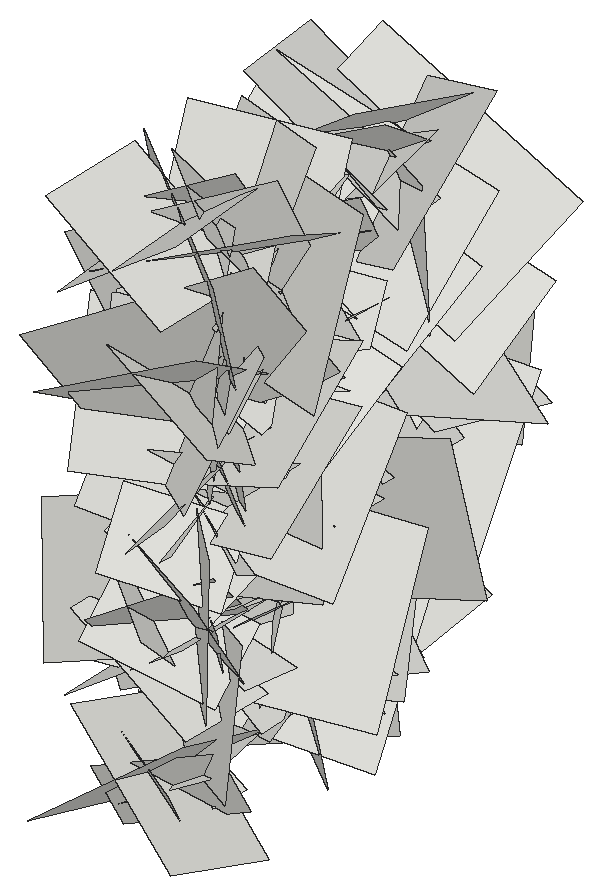
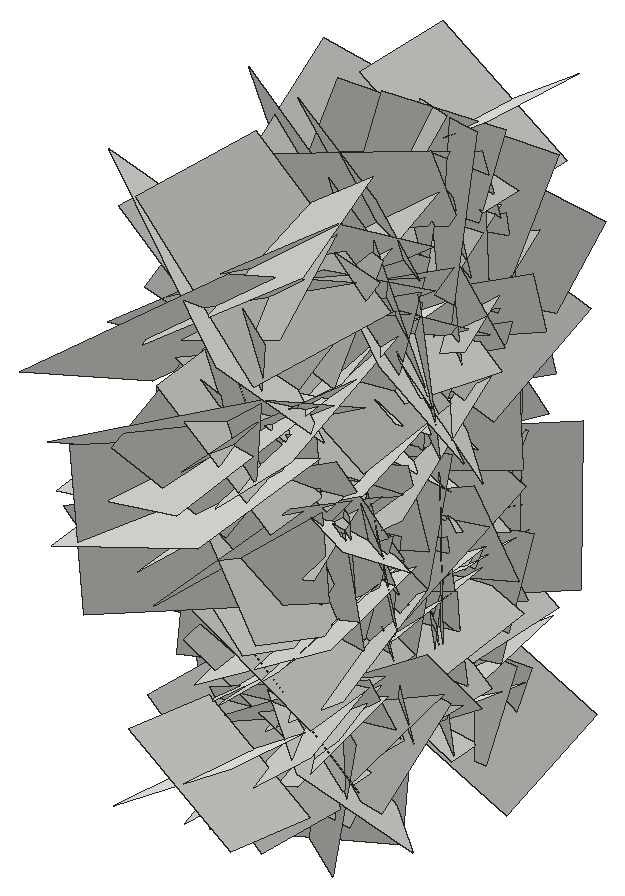
# SketchUp Ruby script. Lengths in inches.
U = 1.inch
M = Sketchup.active_model
def pt(a) = Geom::Point3d.new(a.map { |v| v * U })
def face(e, loops, mat)
  f = e.add_face(loops[0].map { |a| pt(a) })
  loops[1..].each { |l| e.add_face(l.map { |a| pt(a) }).erase! }
  f.material = f.back_material = mat if mat
  f
end
# faces: each face lists its corners as indices into pts; further lists are holes
def faces(e, pts, list, mat = nil) = list.each { |f| face(e, (f[0].is_a?(Array) ? f : [f]).map { |l| l.map { |i| pts[i] } }, mat) }
# xy, xz, yz: faces in a plane at the given z, y or x. An outline is a flat list of corners, or four numbers for a rectangle; further outlines are holes
def ring(l) = l.size == 4 ? [[l[0], l[1]], [l[2], l[1]], [l[2], l[3]], [l[0], l[3]]] : l.each_slice(2).to_a
def flat(e, list, mat, &to3) = list.each { |f| face(e, (f[0].is_a?(Array) ? f : [f]).map { |l| ring(l).map { |u, v| to3.(u, v) } }, mat) }
def xy(e, z, list, mat = nil) = flat(e, list, mat) { |x, y| [x, y, z] }
def xz(e, y, list, mat = nil) = flat(e, list, mat) { |x, z| [x, y, z] }
def yz(e, x, list, mat = nil) = flat(e, list, mat) { |y, z| [x, y, z] }
def lines(e, pts, list) = list.each { |a, b| e.add_line(pt(pts[a]), pt(pts[b])) }
# prism: a flat outline (further loops are holes) pulled along v
def prism(e, loops, v, mat = nil)
  f = face(e, loops, mat); d = Geom::Vector3d.new(v.map { |x| x * U })
  f.pushpull(f.normal.samedirection?(d) ? d.length : -d.length)
end
def box(e, o, s, mat = nil) = prism(e, [[o, [o[0] + s[0], o[1], o[2]], [o[0] + s[0], o[1] + s[1], o[2]], [o[0], o[1] + s[1], o[2]]]], [0, 0, s[2]], mat)
def at(x, y, z, deg = 0) = Geom::Transformation.translation(pt([x, y, z])) * Geom::Transformation.rotation(ORIGIN, Z_AXIS, deg.degrees)
def axes(o, x, y, z) = Geom::Transformation.new([*x, 0, *y, 0, *z, 0, *pt(o).to_a, 1])
def part(name) = M.definitions.add(name)
# library, detail: a bought-in or finely detailed component or shape, given as its bounding box
def library(name, o, s) = part(name).tap { |d| box(d.entities, o, s) }
def detail(e, o, s) = box(e.add_group.entities, o, s)
def put(e, d, t, mat = nil) = e.add_instance(d, t).tap { |i| i.material = mat if mat }
def group(e, t, mat = nil) = e.add_group.tap { |g| g.transformation = t; g.material = mat if mat }.entities
root = M.entities
c1 = part("Component\#6")
p = [[0.01,0,0],[0,3.24,4.54],[4.32,3.24,4.54],[4.33,0,0]]
faces(c1.entities,p,[[0,1,2,3]])
put(root,c1,axes([38.11,185.4,30.76],[0.02152,-0.00963,-1.2106],[0.23963,-1.18945,0.01326],[-1.26071,-0.22625,-0.01814]))
put(root,c1,axes([34.14,183.74,37.84],[0.08456,-0.37494,0.46177],[-0.03825,0.46199,0.38136],[0.62935,0.07846,-0.03886]))
put(root,c1,axes([34.14,188.62,32.29],[-0.0866,-0.74743,0.19758],[-0.06186,0.20408,0.74787],[0.81715,-0.06376,0.07755]))
put(root,c1,axes([34.14,184.65,28.76],[0.04824,-0.62434,-0.28052],[-0.09786,-0.28417,0.61748],[0.7189,0.00321,0.10288]))
put(root,c1,axes([38.11,186.48,30.64],[-0.03295,0.70699,0.47041],[-0.18441,0.45544,-0.69599],[-0.88105,-0.12176,0.12808]))
put(root,c1,axes([38.11,180.55,24.45],[-0.04702,0.95483,-0.28451],[0.08229,-0.28062,-0.95386],[-1.05288,-0.06457,-0.06184]))
put(root,c1,axes([38.11,184.8,33.37],[-0.19651,0.19461,-0.78555],[0.01158,-0.80522,-0.20206],[-0.85778,-0.05545,0.17724]))
put(root,c1,axes([38.11,181.12,36.49],[0.0887,0.85058,-0.45713],[-0.14057,-0.44437,-0.85112],[-1.01388,0.13603,0.07801]))
put(root,c1,axes([34.14,182.11,23.57],[-0.01533,0.32032,-0.55846],[0.07998,-0.55391,-0.31966],[0.67773,0.07262,0.02509]))
put(root,c1,axes([34.14,186.27,36.66],[-0.23271,0.08267,-1.0169],[-0.17131,-1.02986,-0.04883],[1.06781,-0.14721,-0.22945]))
put(root,c1,axes([34.14,181.88,29.24],[0.0732,0.47057,-0.46808],[-0.06498,-0.46407,-0.47558],[0.70054,-0.09222,0.00479]))
put(root,c1,axes([34.14,188.01,25.87],[-0.18323,0.88768,-0.1275],[-0.06793,-0.14175,-0.89995],[0.94816,0.16139,-0.08912]))
put(root,c1,axes([38.11,186.85,26],[-0.04759,0.74401,-0.43208],[-0.09551,-0.43435,-0.73856],[-0.90698,0.0067,0.10045]))
put(root,c1,axes([38.11,182.62,33.52],[0.16113,0.63843,0.91206],[0.00988,0.91976,-0.64538],[-1.18006,0.09488,0.11913]))
put(root,c1,axes([34.14,188.3,31.13],[-0.1103,-0.11339,-0.88165],[-0.13763,-0.87621,0.12802],[0.93214,-0.14279,-0.08543]))
put(root,c1,axes([38.11,182.86,27.86],[-0.00866,0.87216,-0.09866],[-0.12421,-0.09886,-0.86427],[-0.92206,0.00513,0.11735]))
put(root,c1,axes([34.14,188.48,31.6],[0.00806,0.51701,-0.38199],[0.06142,-0.38101,-0.51453],[0.67861,0.02834,0.0511]))
put(root,c1,axes([34.14,189.49,31],[-0.19159,0.03614,-0.77666],[0.1449,-0.78347,-0.06827],[0.81131,0.14846,-0.17121]))
put(root,c1,axes([38.11,186.8,27.07],[0.11611,-1.02809,0.5245],[0.14127,0.5346,1.02006],[-1.21522,-0.03608,0.16869]))
put(root,c1,axes([34.14,181.75,22.9],[0.07496,0.59984,0.04506],[0.05269,0.03939,-0.60235],[0.63545,-0.07402,0.04463]))
put(root,c1,axes([38.11,190.89,25.45],[0.07637,-0.93381,0.1535],[-0.06656,0.14888,0.93522],[-1.00091,-0.08115,-0.05048]))
put(root,c1,axes([38.11,189.24,21.76],[-0.15995,-0.688,0.38857],[0.02017,0.39231,0.70202],[-0.83731,0.14088,-0.05731]))
put(root,c1,axes([34.14,186.9,33.68],[-0.12726,-0.80704,-0.07778],[0.05104,-0.08559,0.81372],[0.85791,-0.11462,-0.05995]))
put(root,c1,axes([34.14,183.3,35.54],[0.06853,-0.0517,0.64839],[0.02911,0.65122,0.04919],[0.68886,-0.02238,-0.06659]))
put(root,c1,axes([38.11,182.91,34.72],[0.14912,-0.41506,0.98502],[0.044,0.99488,0.41329],[-1.13217,-0.016,0.1458]))
put(root,c1,axes([38.11,191.48,24.4],[0.24044,-0.84726,-0.84182],[0.11443,-0.83882,0.87332],[-1.26085,-0.2377,-0.08127]))
put(root,c1,axes([34.14,194.3125,23.26],[-0.02367,-0.75059,-0.08188],[0.02978,-0.08269,0.75031],[0.79979,-0.01914,-0.03036]))
put(root,c1,axes([38.11,189.58,22.99],[0.08755,-0.94666,0.34405],[0.04779,0.34833,0.94763],[-1.06661,-0.0621,0.0707]))
put(root,c1,axes([38.11,183.5625,38.07],[-0.03427,-0.86867,-0.02883],[0.01016,-0.0292,0.8692],[-0.92124,0.03199,0.01066]))
put(root,c1,axes([34.14,186.98,23.44],[-0.07046,0.41434,0.63319],[0.10971,0.63463,-0.40442],[0.79457,-0.05088,0.11199]))
put(root,c1,axes([38.11,186.99,20.26],[-0.04681,-0.17583,0.86867],[0.05724,0.86759,0.17835],[-0.93771,0.06173,-0.03248]))
put(root,c1,axes([34.14,182.78,23.92],[-0.06221,-0.24398,0.83625],[-0.07047,0.83695,0.23952],[0.92069,0.04758,0.07484]))
put(root,c1,axes([38.11,187.32,34.27],[-0.05201,-0.4187,0.7383],[0.02779,0.73844,0.42051],[-0.89926,0.04704,-0.0297]))
put(root,c1,axes([34.14,187.84,31.26],[0.01205,0.8882,0.30464],[-0.22592,0.29915,-0.86424],[0.96935,0.05868,-0.20521]))
put(root,c1,axes([34.14,187.61,26.86],[-0.07932,-0.16974,-0.83453],[-0.0041,-0.83766,0.17072],[0.9027,-0.01872,-0.07255]))
put(root,c1,axes([34.14,184.84,39.1],[0.02023,-0.20369,-0.6632],[0.11732,-0.65406,0.20407],[0.72599,0.11137,-0.0145]))
put(root,c1,axes([38.11,180.54,27.52],[-0.00647,0.86334,-0.00303],[0.00368,-0.003,-0.86336],[-0.91514,-0.00612,-0.00345]))
put(root,c1,axes([38.11,189.53,40.3125],[0.07096,0.70634,-0.4758],[-0.12627,-0.46481,-0.70678],[-0.89387,0.12173,0.06207]))
put(root,c1,axes([38.11,192.58,32.17],[-0.11188,-0.86522,-0.03173],[0.14554,-0.04829,0.85998],[-0.90613,0.09907,0.14204]))
put(root,c1,axes([38.11,185.86,28.71],[0.06844,0.29244,0.76285],[-0.17475,0.75415,-0.27515],[-0.84819,-0.13178,0.11824]))
put(root,c1,axes([34.14,188.23,41.22],[-0.26749,1.02168,-0.17372],[0.00845,-0.17688,-1.05183],[1.0985,0.25014,-0.03421]))
put(root,c1,axes([38.11,187.08,35.11],[0.23629,-0.52338,-1.02054],[0.13084,-1.02265,0.55142],[-1.20867,-0.21302,-0.13982]))
put(root,c1,axes([34.14,187.74,23.43],[-0.08523,-0.9506,0.05636],[-0.09187,0.06363,0.94959],[1.00521,-0.07479,0.09156]))
put(root,c1,axes([34.14,184.52,38.07],[-0.06477,0.36641,0.7198],[0.11209,0.71927,-0.35717],[0.84878,-0.06703,0.10209]))
put(root,c1,axes([34.14,184.92,37.05],[0.01613,-0.13323,-0.78421],[0.01491,-0.78419,0.1335],[0.84304,0.01642,0.01265]))
put(root,c1,axes([38.11,184.92,37.05],[-0.01613,-0.13323,-0.78421],[-0.01491,-0.78419,0.1335],[-0.84304,0.01642,0.01265]))
put(root,c1,axes([38.11,184.52,38.07],[0.06477,0.36641,0.7198],[-0.11209,0.71927,-0.35717],[-0.84878,-0.06703,0.10209]))
put(root,c1,axes([38.11,187.74,23.43],[0.08523,-0.9506,0.05636],[0.09187,0.06363,0.94959],[-1.00521,-0.07479,0.09156]))
put(root,c1,axes([34.14,187.08,35.11],[-0.23629,-0.52338,-1.02054],[-0.13084,-1.02265,0.55142],[1.20867,-0.21302,-0.13982]))
put(root,c1,axes([38.11,188.23,41.22],[0.26749,1.02168,-0.17372],[-0.00845,-0.17688,-1.05183],[-1.0985,0.25014,-0.03421]))
put(root,c1,axes([34.14,185.86,28.71],[-0.06844,0.29244,0.76285],[0.17475,0.75415,-0.27515],[0.84819,-0.13178,0.11824]))
put(root,c1,axes([34.14,192.58,32.17],[0.11188,-0.86522,-0.03173],[-0.14554,-0.04829,0.85998],[0.90613,0.09907,0.14204]))
put(root,c1,axes([34.14,189.53,40.3125],[-0.07096,0.70634,-0.4758],[0.12627,-0.46481,-0.70678],[0.89387,0.12173,0.06207]))
put(root,c1,axes([34.14,180.54,27.52],[0.00647,0.86334,-0.00303],[-0.00368,-0.003,-0.86336],[0.91514,-0.00612,-0.00345]))
put(root,c1,axes([38.11,184.84,39.1],[-0.02023,-0.20369,-0.6632],[-0.11732,-0.65406,0.20407],[-0.72599,0.11137,-0.0145]))
put(root,c1,axes([38.11,187.61,26.86],[0.07932,-0.16974,-0.83453],[0.0041,-0.83766,0.17072],[-0.9027,-0.01872,-0.07255]))
put(root,c1,axes([38.11,187.84,31.26],[-0.01205,0.8882,0.30464],[0.22592,0.29915,-0.86424],[-0.96935,0.05868,-0.20521]))
put(root,c1,axes([34.14,187.32,34.27],[0.05201,-0.4187,0.7383],[-0.02779,0.73844,0.42051],[0.89926,0.04704,-0.0297]))
put(root,c1,axes([38.11,182.78,23.92],[0.06221,-0.24398,0.83625],[0.07047,0.83695,0.23952],[-0.92069,0.04758,0.07484]))
put(root,c1,axes([34.14,186.99,20.26],[0.04681,-0.17583,0.86867],[-0.05724,0.86759,0.17835],[0.93771,0.06173,-0.03248]))
put(root,c1,axes([38.11,186.98,23.44],[0.07046,0.41434,0.63319],[-0.10971,0.63463,-0.40442],[-0.79457,-0.05088,0.11199]))
put(root,c1,axes([34.14,183.5625,38.07],[0.03427,-0.86867,-0.02883],[-0.01016,-0.0292,0.8692],[0.92124,0.03199,0.01066]))
put(root,c1,axes([34.14,189.58,22.99],[-0.08755,-0.94666,0.34405],[-0.04779,0.34833,0.94763],[1.06661,-0.0621,0.0707]))
put(root,c1,axes([38.11,194.3125,23.26],[0.02367,-0.75059,-0.08188],[-0.02978,-0.08269,0.75031],[-0.79979,-0.01914,-0.03036]))
put(root,c1,axes([34.14,191.48,24.4],[-0.24044,-0.84726,-0.84182],[-0.11443,-0.83882,0.87332],[1.26085,-0.2377,-0.08127]))
put(root,c1,axes([34.14,182.91,34.72],[-0.14912,-0.41506,0.98502],[-0.044,0.99488,0.41329],[1.13217,-0.016,0.1458]))
put(root,c1,axes([38.11,183.3,35.54],[-0.06853,-0.0517,0.64839],[-0.02911,0.65122,0.04919],[-0.68886,-0.02238,-0.06659]))
put(root,c1,axes([38.11,186.9,33.68],[0.12726,-0.80704,-0.07778],[-0.05104,-0.08559,0.81372],[-0.85791,-0.11462,-0.05995]))
put(root,c1,axes([34.14,189.24,21.76],[0.15995,-0.688,0.38857],[-0.02017,0.39231,0.70202],[0.83731,0.14088,-0.05731]))
put(root,c1,axes([34.14,190.89,25.45],[-0.07637,-0.93381,0.1535],[0.06656,0.14888,0.93522],[1.00091,-0.08115,-0.05048]))
put(root,c1,axes([38.11,181.75,22.9],[-0.07496,0.59984,0.04506],[-0.05269,0.03939,-0.60235],[-0.63545,-0.07402,0.04463]))
put(root,c1,axes([34.14,186.8,27.07],[-0.11611,-1.02809,0.5245],[-0.14127,0.5346,1.02006],[1.21522,-0.03608,0.16869]))
put(root,c1,axes([38.11,189.49,31],[0.19159,0.03614,-0.77666],[-0.1449,-0.78347,-0.06827],[-0.81131,0.14846,-0.17121]))
put(root,c1,axes([38.11,188.48,31.6],[-0.00806,0.51701,-0.38199],[-0.06142,-0.38101,-0.51453],[-0.67861,0.02834,0.0511]))
put(root,c1,axes([34.14,182.86,27.86],[0.00866,0.87216,-0.09866],[0.12421,-0.09886,-0.86427],[0.92206,0.00513,0.11735]))
put(root,c1,axes([38.11,188.3,31.13],[0.1103,-0.11339,-0.88165],[0.13763,-0.87621,0.12802],[-0.93214,-0.14279,-0.08543]))
put(root,c1,axes([34.14,182.62,33.52],[-0.16113,0.63843,0.91206],[-0.00988,0.91976,-0.64538],[1.18006,0.09488,0.11913]))
put(root,c1,axes([34.14,186.85,26],[0.04759,0.74401,-0.43208],[0.09551,-0.43435,-0.73856],[0.90698,0.0067,0.10045]))
put(root,c1,axes([38.11,188.01,25.87],[0.18323,0.88768,-0.1275],[0.06793,-0.14175,-0.89995],[-0.94816,0.16139,-0.08912]))
put(root,c1,axes([38.11,181.88,29.24],[-0.0732,0.47057,-0.46808],[0.06498,-0.46407,-0.47558],[-0.70054,-0.09222,0.00479]))
put(root,c1,axes([38.11,186.27,36.66],[0.23271,0.08267,-1.0169],[0.17131,-1.02986,-0.04883],[-1.06781,-0.14721,-0.22945]))
put(root,c1,axes([38.11,182.11,23.57],[0.01533,0.32032,-0.55846],[-0.07998,-0.55391,-0.31966],[-0.67773,0.07262,0.02509]))
put(root,c1,axes([34.14,181.12,36.49],[-0.0887,0.85058,-0.45713],[0.14057,-0.44437,-0.85112],[1.01388,0.13603,0.07801]))
put(root,c1,axes([34.14,184.8,33.37],[0.19651,0.19461,-0.78555],[-0.01158,-0.80522,-0.20206],[0.85778,-0.05545,0.17724]))
put(root,c1,axes([34.14,180.55,24.45],[0.04702,0.95483,-0.28451],[-0.08229,-0.28062,-0.95386],[1.05288,-0.06457,-0.06184]))
put(root,c1,axes([34.14,186.48,30.64],[0.03295,0.70699,0.47041],[0.18441,0.45544,-0.69599],[0.88105,-0.12176,0.12808]))
put(root,c1,axes([38.11,184.65,28.76],[-0.04824,-0.62434,-0.28052],[0.09786,-0.28417,0.61748],[-0.7189,0.00321,0.10288]))
put(root,c1,axes([38.11,188.62,32.29],[0.0866,-0.74743,0.19758],[0.06186,0.20408,0.74787],[-0.81715,-0.06376,0.07755]))
put(root,c1,axes([38.11,183.74,37.84],[-0.08456,-0.37494,0.46177],[0.03825,0.46199,0.38136],[-0.62935,0.07846,-0.03886]))
put(root,c1,axes([34.14,185.4,30.76],[-0.02152,-0.00963,-1.2106],[-0.23963,-1.18945,0.01326],[1.26071,-0.22625,-0.01814]))
put(root,c1,axes([34.14,187.18,35.87],[-0.21905,1.32848,-0.23139],[-0.18572,-0.25856,-1.32798],[1.41727,0.17144,-0.20979]))
put(root,c1,axes([38.11,188.41,35.3125],[-0.03073,0.48255,0.4704],[0.10717,0.46862,-0.47449],[-0.70624,0.05011,-0.09248]))
put(root,c1,axes([38.11,183.98,26.9],[0.15473,-0.64925,-0.29626],[-0.07231,-0.3137,0.65387],[-0.75301,-0.10329,-0.12366]))
put(root,c1,axes([38.11,183.4375,30.23],[0.10865,-0.24445,0.66529],[-0.00738,0.67183,0.24793],[-0.75127,-0.04195,0.09378]))
put(root,c1,axes([38.11,185.35,37.93],[0.06077,0.5182,0.40006],[-0.00909,0.40215,-0.51968],[-0.69387,0.04012,0.04185]))
put(root,c1,axes([34.14,182.41,31.86],[-0.21699,-0.67676,1.03332],[0.0082,1.04669,0.68705],[1.3093,-0.11872,0.16695]))
put(root,c1,axes([34.14,181.64,30.57],[0.02444,0.48831,-0.77146],[0.19424,-0.75848,-0.47462],[0.9481,0.1428,0.11713]))
put(root,c1,axes([34.14,184.85,32.98],[-0.15473,1.07562,-0.16592],[0.16403,-0.14519,-1.07739],[1.14193,0.1666,0.13228]))
put(root,c1,axes([38.11,179.78,31.84],[0.01485,0.68647,0.23212],[0.1576,0.2245,-0.67291],[-0.75179,0.06062,-0.13648]))
put(root,c1,axes([38.11,188.93,38.32],[0.06934,0.59373,0.25],[-0.00198,0.25145,-0.59671],[-0.68287,0.05956,0.02711]))
put(root,c1,axes([38.11,193.29,29.97],[-0.02765,-0.60791,0.13872],[0.08921,0.13414,0.60366],[-0.6549,0.04394,0.07638]))
put(root,c1,axes([34.14,189.07,22.99],[0.09993,-0.91741,-0.05408],[0.10319,-0.04408,0.91762],[0.96866,0.09934,-0.09218]))
put(root,c1,axes([34.14,185.63,37.94],[-0.10296,1.07287,0.66666],[-0.13207,0.65722,-1.07584],[1.33238,0.14805,-0.05512]))
put(root,c1,axes([34.14,185.55,26.35],[0.05433,-0.24183,-1.04679],[-0.06418,-1.04696,0.23891],[1.13701,-0.04754,0.0635]))
put(root,c1,axes([38.11,186.02,29.02],[0.12909,0.32312,-0.64935],[0.06195,-0.66067,-0.31779],[-0.76632,0.00102,-0.13508]))
put(root,c1,axes([34.14,190.19,31.82],[0.07854,-1.04848,0.11995],[-0.05802,0.11627,1.05008],[1.11713,0.07975,0.0461]))
put(root,c1,axes([38.11,188.83,29.07],[0.04972,0.59189,0.16701],[0.02122,0.16593,-0.59371],[-0.65156,0.05057,-0.00659]))
put(root,c1,axes([34.14,185.29,39.56],[0.11827,0.82487,-0.51088],[0.03346,-0.51706,-0.82795],[1.02793,-0.07808,0.08573]))
put(root,c1,axes([34.14,186.92,28.87],[0.11772,1.08189,-0.3436],[-0.18933,-0.32428,-1.0788],[1.18826,-0.15885,-0.13785]))
put(root,c1,axes([38.11,191.45,35.51],[0.13227,0.51495,-0.41011],[0.00116,-0.41758,-0.52399],[-0.6978,0.09692,-0.07861]))
put(root,c1,axes([38.11,183.51,30.36],[0.10644,-0.42009,-0.4575],[-0.01901,-0.46521,0.42323],[-0.65811,-0.0545,-0.08622]))
put(root,c1,axes([34.14,184.16,23.6],[0.00632,0.19994,1.20323],[-0.15077,1.19515,-0.1979],[1.28409,0.13934,-0.02916]))
put(root,c1,axes([34.14,189.26,31.29],[0.07003,-0.18149,-1.00879],[0.05402,-1.00905,0.18487],[1.08514,0.06195,0.0559]))
put(root,c1,axes([38.11,191.07,24.72],[0.08022,-0.60182,-0.03468],[0.03515,-0.03074,0.60586],[-0.63802,-0.07736,0.02902]))
put(root,c1,axes([34.14,187.65,25.55],[0.14301,-0.32766,0.90945],[0.11586,0.91755,0.31436],[1.01811,-0.05839,-0.16352]))
put(root,c1,axes([34.14,192.86,38.11],[0.10772,-0.0541,-1.0459],[0.04447,-1.04976,0.05837],[1.10925,0.04734,0.09923]))
put(root,c1,axes([38.11,188.74,27.6],[0.13014,-0.45431,-0.37588],[0.00674,-0.3829,0.46487],[-0.62498,-0.09873,-0.07326]))
put(root,c1,axes([34.14,181.98,27.65],[0.03848,-0.07343,1.06513],[0.13392,1.05855,0.06867],[1.12376,-0.12364,-0.04466]))
put(root,c1,axes([34.14,182.88,33.98],[0.05541,0.90127,0.55592],[0.17138,0.54328,-0.89597],[1.1093,-0.12895,0.11065]))
put(root,c1,axes([34.14,190.1,29],[0.15352,-0.05709,1.12322],[-0.06907,1.13017,0.06585],[1.19015,0.07295,-0.14107]))
put(root,c1,axes([34.14,185.59,36.56],[0.07365,1.00309,0.56692],[0.00038,0.56794,-1.00493],[1.22135,-0.06067,-0.03387]))
put(root,c1,axes([34.14,194.96,38.36],[-0.08597,-0.96025,-0.92678],[-0.03419,-0.92681,0.9631],[1.41421,-0.08078,-0.03305]))
put(root,c1,axes([34.14,188.57,34.3],[-0.02784,1.05016,0.5271],[0.1514,0.52617,-1.0412],[1.23628,-0.04079,0.13938]))
put(root,c1,axes([34.14,186.91,28.91],[-0.08475,0.77289,1.06783],[0.0494,1.07079,-0.77154],[1.39641,0.00903,0.0921]))
put(root,c1,axes([34.14,187.29,32.09],[-0.03087,-0.89426,-0.74249],[0.26998,-0.72958,0.86873],[1.20212,0.14089,-0.21417]))
put(root,c1,axes([34.14,190.5,33.59],[0.11278,1.05886,-0.21225],[0.21462,-0.22906,-1.04119],[1.12442,-0.06248,0.22002]))
put(root,c1,axes([34.14,184.99,36.41],[0.13687,-0.99381,0.45239],[0.15227,0.46704,0.985],[1.14738,0.05657,-0.18469]))
put(root,c1,axes([34.14,181.61,25.33],[-0.14764,0.72138,1.18272],[0.09804,1.19088,-0.71546],[1.46521,-0.007,0.16705]))
put(root,c1,axes([34.14,187.26,33.24],[0.066,-0.95024,-0.64083],[0.19237,-0.6255,0.94515],[1.19957,0.15259,-0.11631]))
put(root,c1,axes([34.14,188.72,38.18],[0.108,1.17484,0.54266],[-0.09899,0.5496,-1.17232],[1.36819,-0.05298,-0.12766]))
put(root,c1,axes([34.14,180.73,30.67],[0.05707,0.69485,1.12415],[-0.04583,1.1254,-0.69356],[1.4001,0.00851,-0.06852]))
put(root,c1,axes([34.14,188.1875,39.24],[0.00053,-0.50504,-1.25708],[0.1621,-1.24903,0.50186],[1.42684,0.14209,-0.05655]))
put(root,c1,axes([34.14,186.51,25.44],[-0.00901,-0.3677,1.34811],[0.26845,1.32541,0.3631],[1.45667,-0.24653,-0.05858]))
put(root,c1,axes([34.14,190.14,35.27],[0.30668,1.10496,-0.445],[0.14325,-0.48543,-1.11748],[1.25452,-0.21469,0.23639]))
